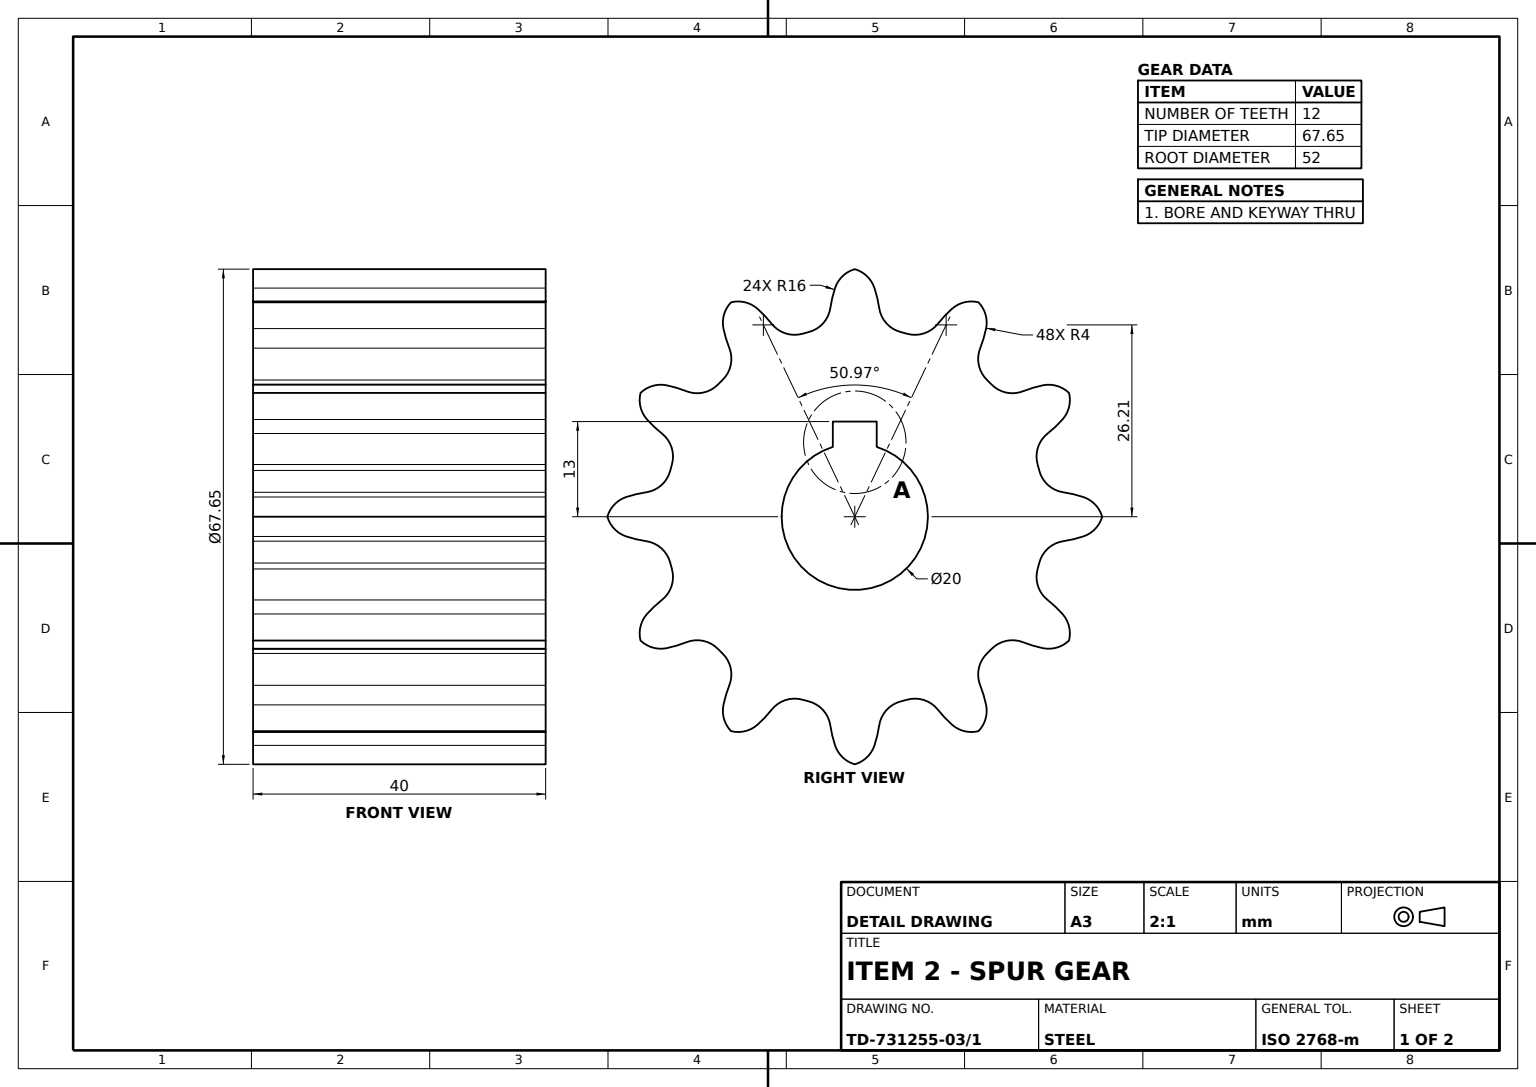
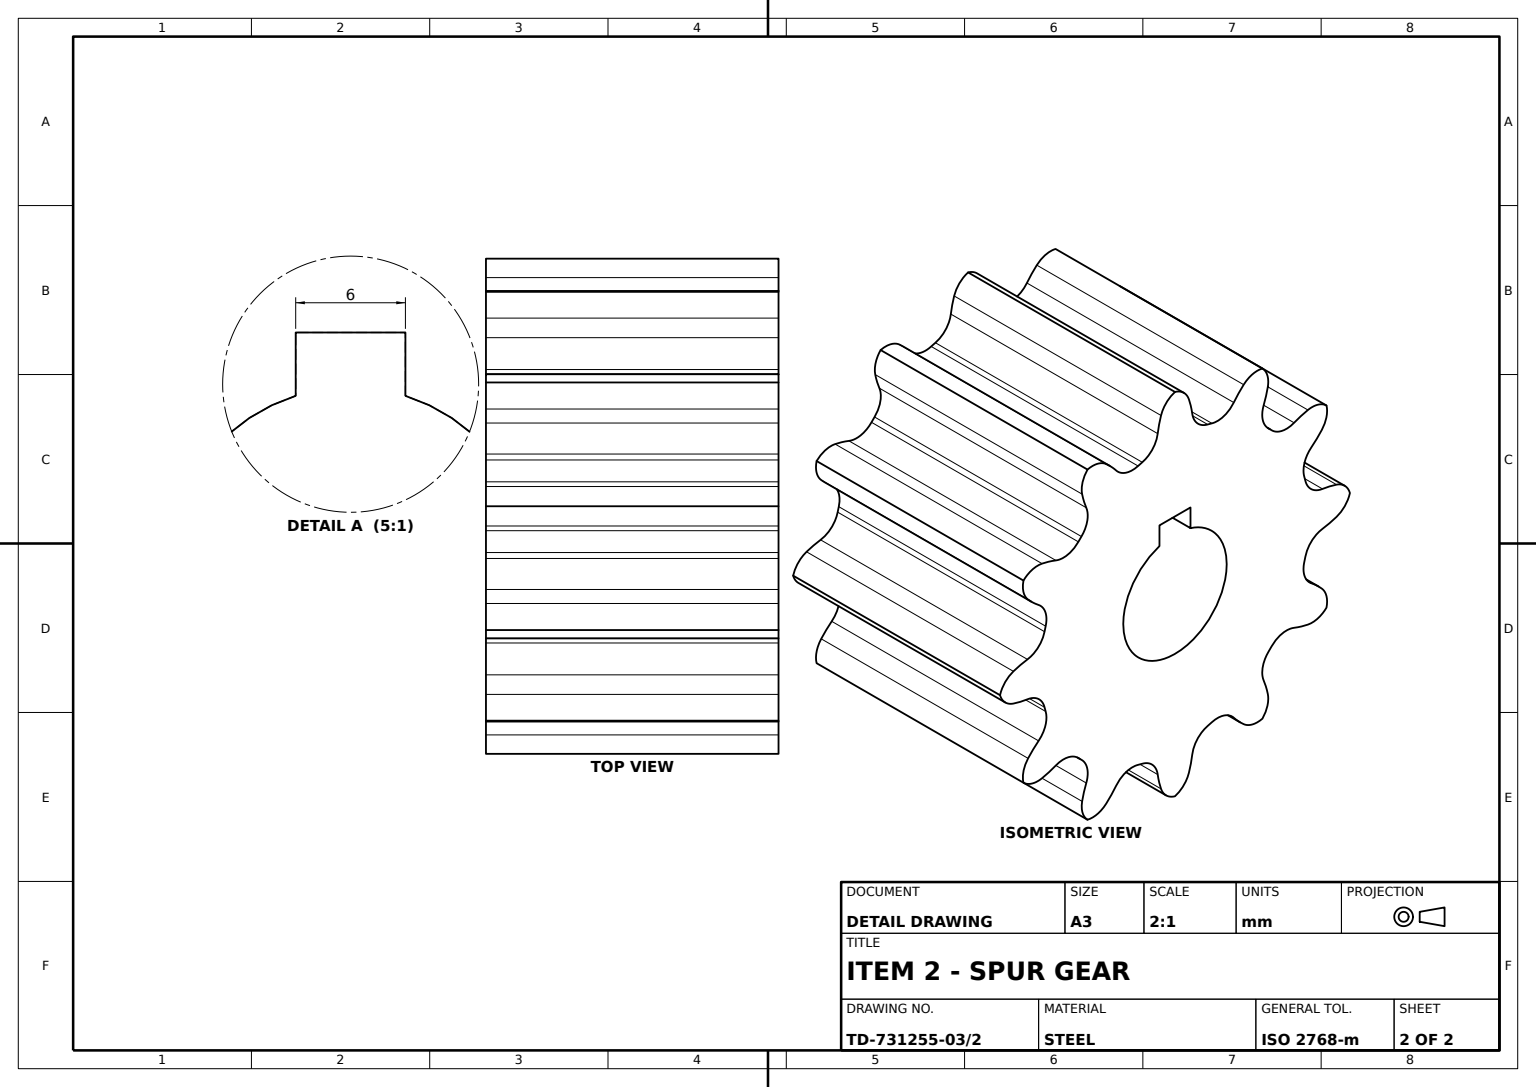
solid
v1 (-11.369537,-26.369339,0)
v2 (-11.369537,-26.369339,40)
e1 v1 v2 LINE
v3 (-7.133298,-25.002321,0)
e2 v3 v1 CIRCLE(AX(P(-8.230729,-28.848832,0),D(0,0,1),D(1,0,0)),4)
v4 (-7.133298,-25.002321,40)
e3 v4 v3 LINE
e4 v2 v4 CIRCLE(AX(P(-8.230729,-28.848832,40),D(0,0,-1),D(1,0,0)),4)
face CYL(AX(P(-8.230729,-28.848832,40),D(0,0,1),D(1,0,0)),4) rev [-e1 -e2 -e3 -e4]
v5 (-17.151749,23.030977,0)
v6 (-17.151749,23.030977,40)
e5 v5 v6 LINE
v7 (-16.868457,21.552436,0)
e6 v7 v5 CIRCLE(AX(P(-20.868457,21.552436,0),D(0,0,1),D(1,0,0)),4)
v8 (-16.868457,21.552436,40)
e7 v7 v8 LINE
e8 v6 v8 CIRCLE(AX(P(-20.868457,21.552436,40),D(0,0,-1),D(1,0,0)),4)
face CYL(AX(P(-20.868457,21.552436,40),D(0,0,1),D(1,0,0)),4) rev [-e5 -e6 e7 -e8]
v9 (-31.236472,2.696073,0)
v10 (-31.236472,2.696073,40)
e9 v9 v10 LINE
v11 (-28.521286,3.338362,40)
e10 v11 v10 CIRCLE(AX(P(-26.209685,-12.493773,40),D(0,0,1),D(1,0,0)),16)
v12 (-28.521286,3.338362,0)
e11 v11 v12 LINE
e12 v12 v9 CIRCLE(AX(P(-26.209685,-12.493773,0),D(0,0,1),D(1,0,0)),16)
face CYL(AX(P(-26.209685,-12.493773,40),D(0,0,-1),D(-1,0,0)),16) [e9 -e10 e11 e12]
v13 (-11.369537,26.369339,40)
v14 (-11.369537,26.369339,0)
e13 v13 v14 LINE
v15 (-7.133298,25.002321,40)
e14 v15 v13 CIRCLE(AX(P(-8.230729,28.848832,40),D(0,0,-1),D(1,0,0)),4)
v16 (-7.133298,25.002321,0)
e15 v16 v15 LINE
e16 v14 v16 CIRCLE(AX(P(-8.230729,28.848832,0),D(0,0,1),D(1,0,0)),4)
face CYL(AX(P(-8.230729,28.848832,40),D(0,0,1),D(1,0,0)),4) rev [-e13 -e14 -e15 -e16]
v17 (11.369537,26.369339,40)
v18 (7.133298,25.002321,40)
e17 v17 v18 CIRCLE(AX(P(8.230729,28.848832,40),D(0,0,-1),D(1,0,0)),4)
v19 (11.369537,26.369339,0)
e18 v19 v17 LINE
v20 (7.133298,25.002321,0)
e19 v20 v19 CIRCLE(AX(P(8.230729,28.848832,0),D(0,0,1),D(1,0,0)),4)
e20 v18 v20 LINE
face CYL(AX(P(8.230729,28.848832,40),D(0,0,1),D(1,0,0)),4) rev [-e17 -e18 -e19 -e20]
v21 (-31.236472,-2.696073,0)
v22 (-33.825155,0,0)
e21 v21 v22 CIRCLE(AX(P(-29.979776,1.101389,0),D(0,0,-1),D(1,0,0)),4)
v23 (-31.236472,-2.696073,40)
e22 v23 v21 LINE
v24 (-33.825155,0,40)
e23 v24 v23 CIRCLE(AX(P(-29.979776,1.101389,40),D(0,0,1),D(1,0,0)),4)
e24 v24 v22 LINE
face CYL(AX(P(-29.979776,1.101389,40),D(0,0,-1),D(-1,0,0)),4) [-e21 -e22 -e23 e24]
v25 (-3,13,40)
v26 (3,13,40)
e25 v25 v26 LINE
v27 (-3,13,0)
e26 v25 v27 LINE
v28 (3,13,0)
e27 v27 v28 LINE
e28 v26 v28 LINE
face PLANE(AX(P(3,13,40),D(0,1,0),D(0,0,1))) rev [-e25 e26 e27 -e28]
v29 (-16.912577,29.293443,40)
v30 (-18.036057,26.513942,40)
e29 v29 v30 CIRCLE(AX(P(-14.036057,26.513942,40),D(0,0,1),D(1,0,0)),4)
v31 (-16.912577,29.293443,0)
e30 v29 v31 LINE
v32 (-18.036057,26.513942,0)
e31 v32 v31 CIRCLE(AX(P(-14.036057,26.513942,0),D(0,0,-1),D(1,0,0)),4)
e32 v30 v32 LINE
face CYL(AX(P(-14.036057,26.513942,40),D(0,0,-1),D(-1,0,0)),4) [-e29 e30 -e31 -e32]
v33 (-28.521286,-3.338362,40)
v34 (-25.219294,-6.323543,40)
e33 v33 v34 CIRCLE(AX(P(-29.099186,-7.296396,40),D(0,0,-1),D(1,0,0)),4)
v35 (-28.521286,-3.338362,0)
e34 v35 v33 LINE
v36 (-25.219294,-6.323543,0)
e35 v36 v35 CIRCLE(AX(P(-29.099186,-7.296396,0),D(0,0,1),D(1,0,0)),4)
e36 v34 v36 LINE
face CYL(AX(P(-29.099186,-7.296396,40),D(0,0,1),D(1,0,0)),4) rev [-e33 -e34 -e35 -e36]
v37 (-24.848832,-8.230729,0)
v38 (-24.848832,-8.230729,40)
e37 v37 v38 LINE
v39 (-25.002321,-7.133298,40)
e38 v39 v38 CIRCLE(AX(P(-28.848832,-8.230729,40),D(0,0,-1),D(1,0,0)),4)
v40 (-25.002321,-7.133298,0)
e39 v40 v39 LINE
e40 v37 v40 CIRCLE(AX(P(-28.848832,-8.230729,0),D(0,0,1),D(1,0,0)),4)
face CYL(AX(P(-28.848832,-8.230729,40),D(0,0,1),D(1,0,0)),4) rev [e37 -e38 -e39 -e40]
v41 (18.085996,-18.678778,0)
v42 (18.678778,-18.085996,0)
e41 v41 v42 CIRCLE(AX(P(0,0,0),D(0,0,1),D(1,0,0)),26)
v43 (18.678778,-18.085996,40)
e42 v42 v43 LINE
v44 (18.085996,-18.678778,40)
e43 v44 v43 CIRCLE(AX(P(0,0,40),D(0,0,1),D(1,0,0)),26)
e44 v44 v41 LINE
face CYL(AX(P(0,0,40),D(0,0,-1),D(-1,0,0)),26) [e41 e42 -e43 e44]
v45 (25.002321,-7.133298,40)
v46 (25.219294,-6.323543,40)
e45 v45 v46 CIRCLE(AX(P(0,0,40),D(0,0,1),D(1,0,0)),26)
v47 (25.002321,-7.133298,0)
e46 v45 v47 LINE
v48 (25.219294,-6.323543,0)
e47 v47 v48 CIRCLE(AX(P(0,0,0),D(0,0,1),D(1,0,0)),26)
e48 v48 v46 LINE
face CYL(AX(P(0,0,40),D(0,0,-1),D(-1,0,0)),26) [-e45 e46 e47 e48]
v49 (-17.953103,-25.703542,0)
v50 (-17.953103,-25.703542,40)
e49 v49 v50 LINE
v51 (-18.036057,-26.513942,0)
e50 v51 v49 CIRCLE(AX(P(-14.036057,-26.513942,0),D(0,0,-1),D(1,0,0)),4)
v52 (-18.036057,-26.513942,40)
e51 v52 v51 LINE
e52 v50 v52 CIRCLE(AX(P(-14.036057,-26.513942,40),D(0,0,1),D(1,0,0)),4)
face CYL(AX(P(-14.036057,-26.513942,40),D(0,0,-1),D(-1,0,0)),4) [-e49 -e50 -e51 -e52]
e53 v21 v35 CIRCLE(AX(P(-26.209685,12.493773,0),D(0,0,1),D(-1,0,0)),16)
e54 v23 v33 CIRCLE(AX(P(-26.209685,12.493773,40),D(0,0,1),D(-1,0,0)),16)
face CYL(AX(P(-26.209685,12.493773,40),D(0,0,-1),D(-1,0,0)),16) [e22 e53 e34 -e54]
v53 (17.151749,-23.030977,0)
e55 v41 v53 CIRCLE(AX(P(20.868457,-21.552436,0),D(0,0,1),D(1,0,0)),4)
v54 (17.151749,-23.030977,40)
e56 v54 v44 CIRCLE(AX(P(20.868457,-21.552436,40),D(0,0,-1),D(1,0,0)),4)
e57 v53 v54 LINE
face CYL(AX(P(20.868457,-21.552436,40),D(0,0,1),D(1,0,0)),4) rev [-e55 -e44 -e56 -e57]
v55 (25.219294,6.323543,40)
v56 (25.219294,6.323543,0)
e58 v55 v56 LINE
v57 (25.002321,7.133298,0)
e59 v56 v57 CIRCLE(AX(P(0,0,0),D(0,0,1),D(1,0,0)),26)
v58 (25.002321,7.133298,40)
e60 v57 v58 LINE
e61 v55 v58 CIRCLE(AX(P(0,0,40),D(0,0,1),D(1,0,0)),26)
face CYL(AX(P(0,0,40),D(0,0,-1),D(-1,0,0)),26) [e58 e59 e60 -e61]
v59 (-17.151749,-23.030977,40)
v60 (-17.151749,-23.030977,0)
e62 v59 v60 LINE
v61 (-16.868457,-21.552436,40)
e63 v61 v59 CIRCLE(AX(P(-20.868457,-21.552436,40),D(0,0,-1),D(1,0,0)),4)
v62 (-16.868457,-21.552436,0)
e64 v62 v61 LINE
e65 v60 v62 CIRCLE(AX(P(-20.868457,-21.552436,0),D(0,0,1),D(1,0,0)),4)
face CYL(AX(P(-20.868457,-21.552436,40),D(0,0,1),D(1,0,0)),4) rev [-e62 -e63 -e64 -e65]
v63 (-6.323543,25.219294,0)
v64 (-3.338362,28.521286,0)
e66 v63 v64 CIRCLE(AX(P(-7.296396,29.099186,0),D(0,0,1),D(1,0,0)),4)
v65 (-6.323543,25.219294,40)
e67 v65 v63 LINE
v66 (-3.338362,28.521286,40)
e68 v66 v65 CIRCLE(AX(P(-7.296396,29.099186,40),D(0,0,-1),D(1,0,0)),4)
e69 v64 v66 LINE
face CYL(AX(P(-7.296396,29.099186,40),D(0,0,1),D(1,0,0)),4) rev [-e66 -e67 -e68 -e69]
e70 v22 v9 CIRCLE(AX(P(-29.979776,-1.101389,0),D(0,0,-1),D(1,0,0)),4)
e71 v10 v24 CIRCLE(AX(P(-29.979776,-1.101389,40),D(0,0,1),D(1,0,0)),4)
face CYL(AX(P(-29.979776,-1.101389,40),D(0,0,-1),D(-1,0,0)),4) [-e70 -e24 -e71 -e9]
v67 (-23.030977,-17.151749,0)
v68 (-23.030977,-17.151749,40)
e72 v67 v68 LINE
v69 (-25.703542,-17.953103,40)
e73 v69 v68 CIRCLE(AX(P(-28.94514,-2.284918,40),D(0,0,1),D(-1,0,0)),16)
v70 (-25.703542,-17.953103,0)
e74 v69 v70 LINE
e75 v70 v67 CIRCLE(AX(P(-28.94514,-2.284918,0),D(0,0,1),D(-1,0,0)),16)
face CYL(AX(P(-28.94514,-2.284918,40),D(0,0,-1),D(-1,0,0)),16) [e72 -e73 e74 e75]
e76 v36 v40 CIRCLE(AX(P(0,0,0),D(0,0,1),D(1,0,0)),26)
e77 v34 v39 CIRCLE(AX(P(0,0,40),D(0,0,1),D(1,0,0)),26)
face CYL(AX(P(0,0,40),D(0,0,-1),D(-1,0,0)),26) [e76 e39 -e77 e36]
v71 (-26.369339,11.369537,40)
v72 (-24.848832,8.230729,40)
e78 v71 v72 CIRCLE(AX(P(-28.848832,8.230729,40),D(0,0,-1),D(1,0,0)),4)
v73 (-26.369339,11.369537,0)
e79 v73 v71 LINE
v74 (-24.848832,8.230729,0)
e80 v74 v73 CIRCLE(AX(P(-28.848832,8.230729,0),D(0,0,1),D(1,0,0)),4)
e81 v74 v72 LINE
face CYL(AX(P(-28.848832,8.230729,40),D(0,0,1),D(1,0,0)),4) rev [-e78 -e79 -e80 e81]
v75 (6.323543,25.219294,0)
e82 v20 v75 CIRCLE(AX(P(0,0,0),D(0,0,1),D(1,0,0)),26)
v76 (6.323543,25.219294,40)
e83 v75 v76 LINE
e84 v18 v76 CIRCLE(AX(P(0,0,40),D(0,0,1),D(1,0,0)),26)
face CYL(AX(P(0,0,40),D(0,0,-1),D(-1,0,0)),26) [e20 e82 e83 -e84]
v77 (-29.412553,-15.943719,0)
v78 (-28.399615,-13.283369,0)
e85 v77 v78 CIRCLE(AX(P(-25.412553,-15.943719,0),D(0,0,-1),D(1,0,0)),4)
v79 (-29.412553,-15.943719,40)
e86 v79 v77 LINE
v80 (-28.399615,-13.283369,40)
e87 v80 v79 CIRCLE(AX(P(-25.412553,-15.943719,40),D(0,0,1),D(1,0,0)),4)
e88 v78 v80 LINE
face CYL(AX(P(-25.412553,-15.943719,40),D(0,0,-1),D(-1,0,0)),4) [-e85 -e86 -e87 -e88]
v81 (-23.030977,17.151749,40)
v82 (-23.030977,17.151749,0)
e89 v81 v82 LINE
v83 (-25.703542,17.953103,0)
e90 v82 v83 CIRCLE(AX(P(-28.94514,2.284918,0),D(0,0,1),D(1,0,0)),16)
v84 (-25.703542,17.953103,40)
e91 v83 v84 LINE
e92 v81 v84 CIRCLE(AX(P(-28.94514,2.284918,40),D(0,0,1),D(1,0,0)),16)
face CYL(AX(P(-28.94514,2.284918,40),D(0,0,-1),D(-1,0,0)),16) [e89 e90 e91 -e92]
v85 (18.678778,18.085996,0)
v86 (23.030977,17.151749,0)
e93 v85 v86 CIRCLE(AX(P(21.552436,20.868457,0),D(0,0,1),D(1,0,0)),4)
v87 (18.678778,18.085996,40)
e94 v87 v85 LINE
v88 (23.030977,17.151749,40)
e95 v88 v87 CIRCLE(AX(P(21.552436,20.868457,40),D(0,0,-1),D(1,0,0)),4)
e96 v86 v88 LINE
face CYL(AX(P(21.552436,20.868457,40),D(0,0,1),D(1,0,0)),4) rev [-e93 -e94 -e95 -e96]
v89 (26.369339,-11.369537,40)
e97 v89 v45 CIRCLE(AX(P(28.848832,-8.230729,40),D(0,0,-1),D(1,0,0)),4)
v90 (26.369339,-11.369537,0)
e98 v90 v89 LINE
e99 v47 v90 CIRCLE(AX(P(28.848832,-8.230729,0),D(0,0,1),D(1,0,0)),4)
face CYL(AX(P(28.848832,-8.230729,40),D(0,0,1),D(1,0,0)),4) rev [-e46 -e97 -e98 -e99]
v91 (-29.293443,16.912577,0)
e100 v91 v83 CIRCLE(AX(P(-26.513942,14.036057,0),D(0,0,-1),D(1,0,0)),4)
v92 (-29.293443,16.912577,40)
e101 v92 v91 LINE
e102 v84 v92 CIRCLE(AX(P(-26.513942,14.036057,40),D(0,0,1),D(1,0,0)),4)
face CYL(AX(P(-26.513942,14.036057,40),D(0,0,-1),D(-1,0,0)),4) [-e100 -e101 -e102 -e91]
v93 (-17.953103,25.703542,40)
e103 v30 v93 CIRCLE(AX(P(-14.036057,26.513942,40),D(0,0,1),D(1,0,0)),4)
v94 (-17.953103,25.703542,0)
e104 v94 v32 CIRCLE(AX(P(-14.036057,26.513942,0),D(0,0,-1),D(1,0,0)),4)
e105 v93 v94 LINE
face CYL(AX(P(-14.036057,26.513942,40),D(0,0,-1),D(-1,0,0)),4) [-e103 e32 -e104 -e105]
v95 (28.399615,-13.283369,40)
e106 v95 v89 CIRCLE(AX(P(16.451367,-23.924768,40),D(0,0,1),D(-1,0,0)),16)
v96 (28.399615,-13.283369,0)
e107 v95 v96 LINE
e108 v96 v90 CIRCLE(AX(P(16.451367,-23.924768,0),D(0,0,1),D(-1,0,0)),16)
face CYL(AX(P(16.451367,-23.924768,40),D(0,0,-1),D(-1,0,0)),16) [-e106 e107 e108 e98]
v97 (26.369339,11.369537,0)
e109 v97 v57 CIRCLE(AX(P(28.848832,8.230729,0),D(0,0,1),D(1,0,0)),4)
v98 (26.369339,11.369537,40)
e110 v98 v97 LINE
e111 v58 v98 CIRCLE(AX(P(28.848832,8.230729,40),D(0,0,-1),D(1,0,0)),4)
face CYL(AX(P(28.848832,8.230729,40),D(0,0,1),D(1,0,0)),4) rev [-e60 -e109 -e110 -e111]
v99 (18.085996,18.678778,0)
e112 v85 v99 CIRCLE(AX(P(0,0,0),D(0,0,1),D(1,0,0)),26)
v100 (18.085996,18.678778,40)
e113 v99 v100 LINE
e114 v87 v100 CIRCLE(AX(P(0,0,40),D(0,0,1),D(1,0,0)),26)
face CYL(AX(P(0,0,40),D(0,0,-1),D(-1,0,0)),26) [e94 e112 e113 -e114]
v101 (17.151749,23.030977,40)
v102 (17.151749,23.030977,0)
e115 v101 v102 LINE
e116 v100 v101 CIRCLE(AX(P(20.868457,21.552436,40),D(0,0,-1),D(1,0,0)),4)
e117 v102 v99 CIRCLE(AX(P(20.868457,21.552436,0),D(0,0,1),D(1,0,0)),4)
face CYL(AX(P(20.868457,21.552436,40),D(0,0,1),D(1,0,0)),4) rev [-e115 -e116 -e113 -e117]
v103 (-6.323543,-25.219294,0)
v104 (-6.323543,-25.219294,40)
e118 v103 v104 LINE
v105 (-3.338362,-28.521286,0)
e119 v105 v103 CIRCLE(AX(P(-7.296396,-29.099186,0),D(0,0,1),D(1,0,0)),4)
v106 (-3.338362,-28.521286,40)
e120 v106 v105 LINE
e121 v104 v106 CIRCLE(AX(P(-7.296396,-29.099186,40),D(0,0,-1),D(1,0,0)),4)
face CYL(AX(P(-7.296396,-29.099186,40),D(0,0,1),D(1,0,0)),4) rev [-e118 -e119 -e120 -e121]
e122 v93 v6 CIRCLE(AX(P(-2.284918,28.94514,40),D(0,0,1),D(-1,0,0)),16)
e123 v94 v5 CIRCLE(AX(P(-2.284918,28.94514,0),D(0,0,1),D(-1,0,0)),16)
face CYL(AX(P(-2.284918,28.94514,40),D(0,0,-1),D(-1,0,0)),16) [-e122 e105 e123 e5]
v107 (17.953103,-25.703542,40)
e124 v107 v54 CIRCLE(AX(P(2.284918,-28.94514,40),D(0,0,1),D(-1,0,0)),16)
v108 (17.953103,-25.703542,0)
e125 v107 v108 LINE
e126 v108 v53 CIRCLE(AX(P(2.284918,-28.94514,0),D(0,0,1),D(-1,0,0)),16)
face CYL(AX(P(2.284918,-28.94514,40),D(0,0,-1),D(-1,0,0)),16) [e57 -e124 e125 e126]
e127 v3 v103 CIRCLE(AX(P(0,0,0),D(0,0,1),D(1,0,0)),26)
e128 v4 v104 CIRCLE(AX(P(0,0,40),D(0,0,1),D(1,0,0)),26)
face CYL(AX(P(0,0,40),D(0,0,-1),D(-1,0,0)),26) [e127 e118 -e128 e3]
v109 (28.521286,3.338362,0)
v110 (28.521286,3.338362,40)
e129 v109 v110 LINE
e130 v56 v109 CIRCLE(AX(P(29.099186,7.296396,0),D(0,0,1),D(1,0,0)),4)
e131 v110 v55 CIRCLE(AX(P(29.099186,7.296396,40),D(0,0,-1),D(1,0,0)),4)
face CYL(AX(P(29.099186,7.296396,40),D(0,0,1),D(1,0,0)),4) rev [-e129 -e130 -e58 -e131]
v111 (33.825155,0,0)
v112 (33.825155,0,40)
e132 v111 v112 LINE
v113 (31.236472,2.696073,0)
e133 v113 v111 CIRCLE(AX(P(29.979776,-1.101389,0),D(0,0,-1),D(1,0,0)),4)
v114 (31.236472,2.696073,40)
e134 v114 v113 LINE
e135 v112 v114 CIRCLE(AX(P(29.979776,-1.101389,40),D(0,0,1),D(1,0,0)),4)
face CYL(AX(P(29.979776,-1.101389,40),D(0,0,-1),D(-1,0,0)),4) [-e132 -e133 -e134 -e135]
v115 (-29.412553,15.943719,40)
e136 v92 v115 CIRCLE(AX(P(-25.412553,15.943719,40),D(0,0,1),D(1,0,0)),4)
v116 (-29.412553,15.943719,0)
e137 v116 v91 CIRCLE(AX(P(-25.412553,15.943719,0),D(0,0,-1),D(1,0,0)),4)
e138 v115 v116 LINE
face CYL(AX(P(-25.412553,15.943719,40),D(0,0,-1),D(-1,0,0)),4) [-e136 e101 -e137 -e138]
v117 (2.696073,-31.236472,0)
v118 (3.338362,-28.521286,0)
e139 v117 v118 CIRCLE(AX(P(-12.493773,-26.209685,0),D(0,0,1),D(-1,0,0)),16)
v119 (3.338362,-28.521286,40)
e140 v118 v119 LINE
v120 (2.696073,-31.236472,40)
e141 v120 v119 CIRCLE(AX(P(-12.493773,-26.209685,40),D(0,0,1),D(-1,0,0)),16)
e142 v120 v117 LINE
face CYL(AX(P(-12.493773,-26.209685,40),D(0,0,-1),D(-1,0,0)),16) [e139 e140 -e141 e142]
v121 (16.912577,29.293443,0)
v122 (16.912577,29.293443,40)
e143 v121 v122 LINE
v123 (17.953103,25.703542,40)
e144 v123 v122 CIRCLE(AX(P(14.036057,26.513942,40),D(0,0,1),D(1,0,0)),4)
v124 (17.953103,25.703542,0)
e145 v124 v123 LINE
e146 v121 v124 CIRCLE(AX(P(14.036057,26.513942,0),D(0,0,-1),D(1,0,0)),4)
face CYL(AX(P(14.036057,26.513942,40),D(0,0,-1),D(-1,0,0)),4) [e143 -e144 -e145 -e146]
v125 (31.236472,-2.696073,40)
e147 v125 v112 CIRCLE(AX(P(29.979776,1.101389,40),D(0,0,1),D(1,0,0)),4)
v126 (31.236472,-2.696073,0)
e148 v126 v125 LINE
e149 v111 v126 CIRCLE(AX(P(29.979776,1.101389,0),D(0,0,-1),D(1,0,0)),4)
face CYL(AX(P(29.979776,1.101389,40),D(0,0,-1),D(-1,0,0)),4) [e132 -e147 -e148 -e149]
v127 (-18.085996,18.678778,0)
v128 (-18.678778,18.085996,0)
e150 v127 v128 CIRCLE(AX(P(0,0,0),D(0,0,1),D(1,0,0)),26)
v129 (-18.678778,18.085996,40)
e151 v128 v129 LINE
v130 (-18.085996,18.678778,40)
e152 v130 v129 CIRCLE(AX(P(0,0,40),D(0,0,1),D(1,0,0)),26)
e153 v130 v127 LINE
face CYL(AX(P(0,0,40),D(0,0,-1),D(-1,0,0)),26) [e150 e151 -e152 e153]
e154 v113 v109 CIRCLE(AX(P(26.209685,-12.493773,0),D(0,0,1),D(-1,0,0)),16)
e155 v114 v110 CIRCLE(AX(P(26.209685,-12.493773,40),D(0,0,1),D(-1,0,0)),16)
face CYL(AX(P(26.209685,-12.493773,40),D(0,0,-1),D(-1,0,0)),16) [e134 e154 e129 -e155]
v131 (-25.002321,7.133298,40)
v132 (-25.002321,7.133298,0)
e156 v131 v132 LINE
e157 v72 v131 CIRCLE(AX(P(-28.848832,8.230729,40),D(0,0,-1),D(1,0,0)),4)
e158 v132 v74 CIRCLE(AX(P(-28.848832,8.230729,0),D(0,0,1),D(1,0,0)),4)
face CYL(AX(P(-28.848832,8.230729,40),D(0,0,1),D(1,0,0)),4) rev [-e156 -e157 -e81 -e158]
v133 (-16.912577,-29.293443,40)
e159 v52 v133 CIRCLE(AX(P(-14.036057,-26.513942,40),D(0,0,1),D(1,0,0)),4)
v134 (-16.912577,-29.293443,0)
e160 v134 v51 CIRCLE(AX(P(-14.036057,-26.513942,0),D(0,0,-1),D(1,0,0)),4)
e161 v133 v134 LINE
face CYL(AX(P(-14.036057,-26.513942,40),D(0,0,-1),D(-1,0,0)),4) [-e159 e51 -e160 -e161]
v135 (-18.678778,-18.085996,0)
v136 (-18.085996,-18.678778,0)
e162 v135 v136 CIRCLE(AX(P(0,0,0),D(0,0,1),D(1,0,0)),26)
v137 (-18.085996,-18.678778,40)
e163 v136 v137 LINE
v138 (-18.678778,-18.085996,40)
e164 v138 v137 CIRCLE(AX(P(0,0,40),D(0,0,1),D(1,0,0)),26)
e165 v138 v135 LINE
face CYL(AX(P(0,0,40),D(0,0,-1),D(-1,0,0)),26) [e162 e163 -e164 e165]
v139 (13.283369,-28.399615,0)
v140 (13.283369,-28.399615,40)
e166 v139 v140 LINE
v141 (16.912577,-29.293443,0)
e167 v141 v139 CIRCLE(AX(P(15.943719,-25.412553,0),D(0,0,-1),D(1,0,0)),4)
v142 (16.912577,-29.293443,40)
e168 v141 v142 LINE
e169 v140 v142 CIRCLE(AX(P(15.943719,-25.412553,40),D(0,0,1),D(1,0,0)),4)
face CYL(AX(P(15.943719,-25.412553,40),D(0,0,-1),D(-1,0,0)),4) [-e166 -e167 e168 -e169]
v143 (2.696073,31.236472,0)
v144 (2.696073,31.236472,40)
e170 v143 v144 LINE
v145 (3.338362,28.521286,40)
e171 v145 v144 CIRCLE(AX(P(-12.493773,26.209685,40),D(0,0,1),D(1,0,0)),16)
v146 (3.338362,28.521286,0)
e172 v145 v146 LINE
e173 v146 v143 CIRCLE(AX(P(-12.493773,26.209685,0),D(0,0,1),D(1,0,0)),16)
face CYL(AX(P(-12.493773,26.209685,40),D(0,0,-1),D(-1,0,0)),16) [e170 -e171 e172 e173]
v147 (23.030977,-17.151749,0)
e174 v147 v42 CIRCLE(AX(P(21.552436,-20.868457,0),D(0,0,1),D(1,0,0)),4)
v148 (23.030977,-17.151749,40)
e175 v148 v147 LINE
e176 v43 v148 CIRCLE(AX(P(21.552436,-20.868457,40),D(0,0,-1),D(1,0,0)),4)
face CYL(AX(P(21.552436,-20.868457,40),D(0,0,1),D(1,0,0)),4) rev [-e174 -e175 -e176 -e42]
v149 (-25.219294,6.323543,0)
e177 v132 v149 CIRCLE(AX(P(0,0,0),D(0,0,1),D(1,0,0)),26)
v150 (-25.219294,6.323543,40)
e178 v149 v150 LINE
e179 v131 v150 CIRCLE(AX(P(0,0,40),D(0,0,1),D(1,0,0)),26)
face CYL(AX(P(0,0,40),D(0,0,-1),D(-1,0,0)),26) [e156 e177 e178 -e179]
v151 (25.703542,17.953103,40)
v152 (25.703542,17.953103,0)
e180 v151 v152 LINE
v153 (29.293443,16.912577,40)
e181 v153 v151 CIRCLE(AX(P(26.513942,14.036057,40),D(0,0,1),D(1,0,0)),4)
v154 (29.293443,16.912577,0)
e182 v154 v153 LINE
e183 v152 v154 CIRCLE(AX(P(26.513942,14.036057,0),D(0,0,-1),D(1,0,0)),4)
face CYL(AX(P(26.513942,14.036057,40),D(0,0,-1),D(-1,0,0)),4) [-e180 -e181 -e182 -e183]
e184 v76 v145 CIRCLE(AX(P(7.296396,29.099186,40),D(0,0,-1),D(1,0,0)),4)
e185 v146 v75 CIRCLE(AX(P(7.296396,29.099186,0),D(0,0,1),D(1,0,0)),4)
face CYL(AX(P(7.296396,29.099186,40),D(0,0,1),D(1,0,0)),4) rev [-e184 -e83 -e185 -e172]
v155 (-28.399615,13.283369,40)
e186 v155 v71 CIRCLE(AX(P(-16.451367,23.924768,40),D(0,0,1),D(-1,0,0)),16)
v156 (-28.399615,13.283369,0)
e187 v155 v156 LINE
e188 v156 v73 CIRCLE(AX(P(-16.451367,23.924768,0),D(0,0,1),D(-1,0,0)),16)
face CYL(AX(P(-16.451367,23.924768,40),D(0,0,-1),D(-1,0,0)),16) [e79 -e186 e187 e188]
e189 v152 v86 CIRCLE(AX(P(28.94514,2.284918,0),D(0,0,1),D(-1,0,0)),16)
e190 v151 v88 CIRCLE(AX(P(28.94514,2.284918,40),D(0,0,1),D(-1,0,0)),16)
face CYL(AX(P(28.94514,2.284918,40),D(0,0,-1),D(-1,0,0)),16) [e180 e189 e96 -e190]
v157 (28.399615,13.283369,0)
v158 (28.399615,13.283369,40)
e191 v157 v158 LINE
e192 v154 v157 CIRCLE(AX(P(25.412553,15.943719,0),D(0,0,-1),D(1,0,0)),4)
e193 v158 v153 CIRCLE(AX(P(25.412553,15.943719,40),D(0,0,1),D(1,0,0)),4)
face CYL(AX(P(25.412553,15.943719,40),D(0,0,-1),D(-1,0,0)),4) [-e191 -e192 e182 -e193]
e194 v129 v81 CIRCLE(AX(P(-21.552436,20.868457,40),D(0,0,-1),D(1,0,0)),4)
e195 v82 v128 CIRCLE(AX(P(-21.552436,20.868457,0),D(0,0,1),D(1,0,0)),4)
face CYL(AX(P(-21.552436,20.868457,40),D(0,0,1),D(1,0,0)),4) rev [-e89 -e194 -e151 -e195]
e196 v135 v67 CIRCLE(AX(P(-21.552436,-20.868457,0),D(0,0,1),D(1,0,0)),4)
e197 v68 v138 CIRCLE(AX(P(-21.552436,-20.868457,40),D(0,0,-1),D(1,0,0)),4)
face CYL(AX(P(-21.552436,-20.868457,40),D(0,0,1),D(1,0,0)),4) rev [-e72 -e196 -e165 -e197]
v159 (-3,9.539392,0)
e198 v159 v27 LINE
v160 (-3,9.539392,40)
e199 v160 v25 LINE
e200 v160 v159 LINE
face PLANE(AX(P(-3,9.539392,40),D(-1,0,0),D(0,0,1))) rev [e198 -e26 -e199 e200]
v161 (6.323543,-25.219294,0)
e201 v161 v118 CIRCLE(AX(P(7.296396,-29.099186,0),D(0,0,1),D(1,0,0)),4)
v162 (6.323543,-25.219294,40)
e202 v162 v161 LINE
e203 v119 v162 CIRCLE(AX(P(7.296396,-29.099186,40),D(0,0,-1),D(1,0,0)),4)
face CYL(AX(P(7.296396,-29.099186,40),D(0,0,1),D(1,0,0)),4) rev [-e201 -e202 -e203 -e140]
e204 v65 v15 CIRCLE(AX(P(0,0,40),D(0,0,1),D(1,0,0)),26)
e205 v63 v16 CIRCLE(AX(P(0,0,0),D(0,0,1),D(1,0,0)),26)
face CYL(AX(P(0,0,40),D(0,0,-1),D(-1,0,0)),26) [e15 -e204 e67 e205]
v163 (3,9.539392,40)
e206 v26 v163 LINE
v164 (10,0,40)
e207 v163 v164 CIRCLE(AX(P(0,0,40),D(0,0,-1),D(-1,0,0)),10)
v165 (-10,0,40)
e208 v164 v165 CIRCLE(AX(P(0,0,40),D(0,0,-1),D(-1,0,0)),10)
e209 v165 v160 CIRCLE(AX(P(0,0,40),D(0,0,-1),D(-1,0,0)),10)
v166 (13.283369,28.399615,40)
e210 v166 v17 CIRCLE(AX(P(23.924768,16.451367,40),D(0,0,1),D(-1,0,0)),16)
v167 (0,33.825155,40)
e211 v144 v167 CIRCLE(AX(P(-1.101389,29.979776,40),D(0,0,1),D(1,0,0)),4)
v168 (-2.696073,31.236472,40)
e212 v167 v168 CIRCLE(AX(P(1.101389,29.979776,40),D(0,0,1),D(1,0,0)),4)
e213 v168 v66 CIRCLE(AX(P(12.493773,26.209685,40),D(0,0,1),D(-1,0,0)),16)
v169 (-13.283369,28.399615,40)
e214 v13 v169 CIRCLE(AX(P(-23.924768,16.451367,40),D(0,0,1),D(1,0,0)),16)
e215 v169 v29 CIRCLE(AX(P(-15.943719,25.412553,40),D(0,0,1),D(1,0,0)),4)
e216 v8 v130 CIRCLE(AX(P(-20.868457,21.552436,40),D(0,0,-1),D(1,0,0)),4)
e217 v115 v155 CIRCLE(AX(P(-25.412553,15.943719,40),D(0,0,1),D(1,0,0)),4)
e218 v150 v11 CIRCLE(AX(P(-29.099186,7.296396,40),D(0,0,-1),D(1,0,0)),4)
v170 (-26.369339,-11.369537,40)
e219 v38 v170 CIRCLE(AX(P(-28.848832,-8.230729,40),D(0,0,-1),D(1,0,0)),4)
e220 v170 v80 CIRCLE(AX(P(-16.451367,-23.924768,40),D(0,0,1),D(1,0,0)),16)
v171 (-29.293443,-16.912577,40)
e221 v79 v171 CIRCLE(AX(P(-25.412553,-15.943719,40),D(0,0,1),D(1,0,0)),4)
e222 v171 v69 CIRCLE(AX(P(-26.513942,-14.036057,40),D(0,0,1),D(1,0,0)),4)
e223 v137 v61 CIRCLE(AX(P(-20.868457,-21.552436,40),D(0,0,-1),D(1,0,0)),4)
e224 v59 v50 CIRCLE(AX(P(-2.284918,-28.94514,40),D(0,0,1),D(1,0,0)),16)
v172 (-13.283369,-28.399615,40)
e225 v133 v172 CIRCLE(AX(P(-15.943719,-25.412553,40),D(0,0,1),D(1,0,0)),4)
e226 v172 v2 CIRCLE(AX(P(-23.924768,-16.451367,40),D(0,0,1),D(-1,0,0)),16)
v173 (-2.696073,-31.236472,40)
e227 v106 v173 CIRCLE(AX(P(12.493773,-26.209685,40),D(0,0,1),D(1,0,0)),16)
v174 (0,-33.825155,40)
e228 v173 v174 CIRCLE(AX(P(1.101389,-29.979776,40),D(0,0,1),D(1,0,0)),4)
e229 v174 v120 CIRCLE(AX(P(-1.101389,-29.979776,40),D(0,0,1),D(1,0,0)),4)
v175 (7.133298,-25.002321,40)
e230 v162 v175 CIRCLE(AX(P(0,0,40),D(0,0,1),D(1,0,0)),26)
v176 (11.369537,-26.369339,40)
e231 v175 v176 CIRCLE(AX(P(8.230729,-28.848832,40),D(0,0,-1),D(1,0,0)),4)
e232 v176 v140 CIRCLE(AX(P(23.924768,-16.451367,40),D(0,0,1),D(1,0,0)),16)
e233 v142 v107 CIRCLE(AX(P(14.036057,-26.513942,40),D(0,0,1),D(1,0,0)),4)
v177 (25.703542,-17.953103,40)
e234 v148 v177 CIRCLE(AX(P(28.94514,-2.284918,40),D(0,0,1),D(1,0,0)),16)
v178 (29.293443,-16.912577,40)
e235 v177 v178 CIRCLE(AX(P(26.513942,-14.036057,40),D(0,0,1),D(1,0,0)),4)
e236 v178 v95 CIRCLE(AX(P(25.412553,-15.943719,40),D(0,0,1),D(1,0,0)),4)
v179 (28.521286,-3.338362,40)
e237 v46 v179 CIRCLE(AX(P(29.099186,-7.296396,40),D(0,0,-1),D(1,0,0)),4)
e238 v179 v125 CIRCLE(AX(P(26.209685,12.493773,40),D(0,0,1),D(1,0,0)),16)
e239 v98 v158 CIRCLE(AX(P(16.451367,23.924768,40),D(0,0,1),D(1,0,0)),16)
e240 v101 v123 CIRCLE(AX(P(2.284918,28.94514,40),D(0,0,1),D(1,0,0)),16)
e241 v122 v166 CIRCLE(AX(P(15.943719,25.412553,40),D(0,0,1),D(1,0,0)),4)
face PLANE(AX(P(-6.246887,13.104843,40),D(0,0,1),D(1,0,0))) [e206 e207 e208 e209 e199 e25] [e210 e17 e84 e184 e171 e211 e212 e213 e68 e204 e14 e214 e215 e29 e103 e122 e8 e216 e152 e194 e92 e102 e136 e217 e186 e78 e157 e179 e218 e10 e71 e23 e54 e33 e77 e38 e219 e220 e87 e221 e222 e73 e197 e164 e223 e63 e224 e52 e159 e225 e226 e4 e128 e121 e227 e228 e229 e141 e203 e230 e231 e232 e169 e233 e124 e56 e43 e176 e234 e235 e236 e106 e97 e45 e237 e238 e147 e135 e155 e131 e61 e111 e239 e193 e181 e190 e95 e114 e116 e240 e144 e241]
v180 (0,33.825155,0)
e242 v180 v143 CIRCLE(AX(P(-1.101389,29.979776,0),D(0,0,-1),D(1,0,0)),4)
e243 v167 v180 LINE
face CYL(AX(P(-1.101389,29.979776,40),D(0,0,-1),D(-1,0,0)),4) [-e242 -e243 -e211 -e170]
v181 (-2.696073,31.236472,0)
e244 v181 v64 CIRCLE(AX(P(12.493773,26.209685,0),D(0,0,1),D(-1,0,0)),16)
e245 v168 v181 LINE
face CYL(AX(P(12.493773,26.209685,40),D(0,0,-1),D(-1,0,0)),16) [e244 e69 -e213 e245]
v182 (28.521286,-3.338362,0)
e246 v179 v182 LINE
e247 v182 v126 CIRCLE(AX(P(26.209685,12.493773,0),D(0,0,1),D(1,0,0)),16)
face CYL(AX(P(26.209685,12.493773,40),D(0,0,-1),D(-1,0,0)),16) [-e238 e246 e247 e148]
e248 v62 v136 CIRCLE(AX(P(-20.868457,-21.552436,0),D(0,0,1),D(1,0,0)),4)
face CYL(AX(P(-20.868457,-21.552436,40),D(0,0,1),D(1,0,0)),4) rev [-e248 e64 -e223 -e163]
e249 v156 v116 CIRCLE(AX(P(-25.412553,15.943719,0),D(0,0,-1),D(1,0,0)),4)
face CYL(AX(P(-25.412553,15.943719,40),D(0,0,-1),D(-1,0,0)),4) [-e249 -e187 -e217 e138]
v183 (29.293443,-16.912577,0)
e250 v183 v178 LINE
e251 v96 v183 CIRCLE(AX(P(25.412553,-15.943719,0),D(0,0,-1),D(1,0,0)),4)
face CYL(AX(P(25.412553,-15.943719,40),D(0,0,-1),D(-1,0,0)),4) [-e107 -e236 -e250 -e251]
v184 (7.133298,-25.002321,0)
e252 v184 v175 LINE
v185 (11.369537,-26.369339,0)
e253 v185 v184 CIRCLE(AX(P(8.230729,-28.848832,0),D(0,0,1),D(1,0,0)),4)
e254 v176 v185 LINE
face CYL(AX(P(8.230729,-28.848832,40),D(0,0,1),D(1,0,0)),4) rev [-e231 -e252 -e253 -e254]
v186 (-2.696073,-31.236472,0)
e255 v186 v173 LINE
v187 (0,-33.825155,0)
e256 v187 v186 CIRCLE(AX(P(1.101389,-29.979776,0),D(0,0,-1),D(1,0,0)),4)
e257 v174 v187 LINE
face CYL(AX(P(1.101389,-29.979776,40),D(0,0,-1),D(-1,0,0)),4) [-e255 -e256 -e257 -e228]
v188 (25.703542,-17.953103,0)
e258 v147 v188 CIRCLE(AX(P(28.94514,-2.284918,0),D(0,0,1),D(1,0,0)),16)
e259 v188 v177 LINE
face CYL(AX(P(28.94514,-2.284918,40),D(0,0,-1),D(-1,0,0)),16) [e258 e259 -e234 e175]
v189 (-13.283369,-28.399615,0)
e260 v172 v189 LINE
e261 v189 v1 CIRCLE(AX(P(-23.924768,-16.451367,0),D(0,0,1),D(-1,0,0)),16)
face CYL(AX(P(-23.924768,-16.451367,40),D(0,0,-1),D(-1,0,0)),16) [e1 -e226 e260 e261]
v190 (3,9.539392,0)
e262 v28 v190 LINE
e263 v163 v190 LINE
face PLANE(AX(P(3,9.539392,40),D(1,0,0),D(0,0,-1))) rev [-e206 e28 e262 -e263]
v191 (-26.369339,-11.369537,0)
e264 v170 v191 LINE
e265 v191 v37 CIRCLE(AX(P(-28.848832,-8.230729,0),D(0,0,1),D(1,0,0)),4)
face CYL(AX(P(-28.848832,-8.230729,40),D(0,0,1),D(1,0,0)),4) rev [-e264 -e219 -e37 -e265]
v192 (-13.283369,28.399615,0)
e266 v14 v192 CIRCLE(AX(P(-23.924768,16.451367,0),D(0,0,1),D(1,0,0)),16)
e267 v192 v169 LINE
face CYL(AX(P(-23.924768,16.451367,40),D(0,0,-1),D(-1,0,0)),16) [e266 e267 -e214 e13]
v193 (13.283369,28.399615,0)
e268 v193 v19 CIRCLE(AX(P(23.924768,16.451367,0),D(0,0,1),D(-1,0,0)),16)
e269 v166 v193 LINE
face CYL(AX(P(23.924768,16.451367,40),D(0,0,-1),D(-1,0,0)),16) [e268 e18 -e210 e269]
e270 v97 v157 CIRCLE(AX(P(16.451367,23.924768,0),D(0,0,1),D(1,0,0)),16)
face CYL(AX(P(16.451367,23.924768,40),D(0,0,-1),D(-1,0,0)),16) [e270 e191 -e239 e110]
e271 v31 v192 CIRCLE(AX(P(-15.943719,25.412553,0),D(0,0,-1),D(1,0,0)),4)
face CYL(AX(P(-15.943719,25.412553,40),D(0,0,-1),D(-1,0,0)),4) [-e30 -e215 -e267 -e271]
e272 v189 v134 CIRCLE(AX(P(-15.943719,-25.412553,0),D(0,0,-1),D(1,0,0)),4)
face CYL(AX(P(-15.943719,-25.412553,40),D(0,0,-1),D(-1,0,0)),4) [-e225 e161 -e272 -e260]
e273 v191 v78 CIRCLE(AX(P(-16.451367,-23.924768,0),D(0,0,1),D(1,0,0)),16)
face CYL(AX(P(-16.451367,-23.924768,40),D(0,0,-1),D(-1,0,0)),16) [e88 -e220 e264 e273]
e274 v181 v180 CIRCLE(AX(P(1.101389,29.979776,0),D(0,0,-1),D(1,0,0)),4)
face CYL(AX(P(1.101389,29.979776,40),D(0,0,-1),D(-1,0,0)),4) [-e274 -e245 -e212 e243]
e275 v183 v188 CIRCLE(AX(P(26.513942,-14.036057,0),D(0,0,-1),D(1,0,0)),4)
face CYL(AX(P(26.513942,-14.036057,40),D(0,0,-1),D(-1,0,0)),4) [e250 -e235 -e259 -e275]
e276 v182 v48 CIRCLE(AX(P(29.099186,-7.296396,0),D(0,0,1),D(1,0,0)),4)
face CYL(AX(P(29.099186,-7.296396,40),D(0,0,1),D(1,0,0)),4) rev [-e246 -e237 -e48 -e276]
e277 v127 v7 CIRCLE(AX(P(-20.868457,21.552436,0),D(0,0,1),D(1,0,0)),4)
face CYL(AX(P(-20.868457,21.552436,40),D(0,0,1),D(1,0,0)),4) rev [-e216 -e7 -e277 -e153]
e278 v102 v124 CIRCLE(AX(P(2.284918,28.94514,0),D(0,0,1),D(1,0,0)),16)
face CYL(AX(P(2.284918,28.94514,40),D(0,0,-1),D(-1,0,0)),16) [e278 e145 -e240 e115]
v194 (10,0,0)
v195 (-10,0,0)
e279 v194 v195 CIRCLE(AX(P(0,0,0),D(0,0,-1),D(-1,0,0)),10)
e280 v165 v195 LINE
e281 v164 v194 LINE
face CYL(AX(P(0,0,40),D(0,0,-1),D(-1,0,0)),10) rev [e279 -e280 -e208 e281]
v196 (-29.293443,-16.912577,0)
e282 v70 v196 CIRCLE(AX(P(-26.513942,-14.036057,0),D(0,0,-1),D(1,0,0)),4)
e283 v171 v196 LINE
face CYL(AX(P(-26.513942,-14.036057,40),D(0,0,-1),D(-1,0,0)),4) [-e282 -e74 -e222 e283]
e284 v161 v184 CIRCLE(AX(P(0,0,0),D(0,0,1),D(1,0,0)),26)
face CYL(AX(P(0,0,40),D(0,0,-1),D(-1,0,0)),26) [-e230 e202 e284 e252]
e285 v185 v139 CIRCLE(AX(P(23.924768,-16.451367,0),D(0,0,1),D(1,0,0)),16)
face CYL(AX(P(23.924768,-16.451367,40),D(0,0,-1),D(-1,0,0)),16) [e166 -e232 e254 e285]
e286 v190 v194 CIRCLE(AX(P(0,0,0),D(0,0,-1),D(-1,0,0)),10)
face CYL(AX(P(0,0,40),D(0,0,-1),D(-1,0,0)),10) rev [e263 e286 -e281 -e207]
e287 v12 v149 CIRCLE(AX(P(-29.099186,7.296396,0),D(0,0,1),D(1,0,0)),4)
face CYL(AX(P(-29.099186,7.296396,40),D(0,0,1),D(1,0,0)),4) rev [-e218 -e178 -e287 -e11]
e288 v108 v141 CIRCLE(AX(P(14.036057,-26.513942,0),D(0,0,-1),D(1,0,0)),4)
face CYL(AX(P(14.036057,-26.513942,40),D(0,0,-1),D(-1,0,0)),4) [-e125 -e233 -e168 -e288]
e289 v105 v186 CIRCLE(AX(P(12.493773,-26.209685,0),D(0,0,1),D(1,0,0)),16)
face CYL(AX(P(12.493773,-26.209685,40),D(0,0,-1),D(-1,0,0)),16) [e255 -e227 e120 e289]
e290 v193 v121 CIRCLE(AX(P(15.943719,25.412553,0),D(0,0,-1),D(1,0,0)),4)
face CYL(AX(P(15.943719,25.412553,40),D(0,0,-1),D(-1,0,0)),4) [-e290 -e269 -e241 -e143]
e291 v60 v49 CIRCLE(AX(P(-2.284918,-28.94514,0),D(0,0,1),D(1,0,0)),16)
face CYL(AX(P(-2.284918,-28.94514,40),D(0,0,-1),D(-1,0,0)),16) [-e224 e62 e291 e49]
e292 v195 v159 CIRCLE(AX(P(0,0,0),D(0,0,-1),D(-1,0,0)),10)
face CYL(AX(P(0,0,40),D(0,0,-1),D(-1,0,0)),10) rev [-e209 e280 e292 -e200]
e293 v196 v77 CIRCLE(AX(P(-25.412553,-15.943719,0),D(0,0,-1),D(1,0,0)),4)
face CYL(AX(P(-25.412553,-15.943719,40),D(0,0,-1),D(-1,0,0)),4) [e86 -e293 -e283 -e221]
e294 v117 v187 CIRCLE(AX(P(-1.101389,-29.979776,0),D(0,0,-1),D(1,0,0)),4)
face CYL(AX(P(-1.101389,-29.979776,40),D(0,0,-1),D(-1,0,0)),4) [-e294 -e142 -e229 e257]
face PLANE(AX(P(-6.246887,13.104843,0),D(0,0,1),D(1,0,0))) rev [-e27 -e198 -e292 -e279 -e286 -e262] [e119 -e127 e2 -e261 e272 e160 e50 -e291 e65 e248 -e162 e196 -e75 e282 e293 e85 -e273 e265 e40 -e76 e35 -e53 e21 e70 -e12 e287 -e177 e158 e80 -e188 e249 e137 e100 -e90 e195 -e150 e277 e6 -e123 e104 e31 e271 -e266 e16 -e205 e66 -e244 e274 e242 -e173 e185 -e82 e19 -e268 e290 e146 -e278 e117 -e112 e93 -e189 e183 e192 -e270 e109 -e59 e130 -e154 e133 e149 -e247 e276 -e47 e99 -e108 e251 e275 -e258 e174 -e41 e55 -e126 e288 e167 -e285 e253 -e284 e201 -e139 e294 e256 -e289]
